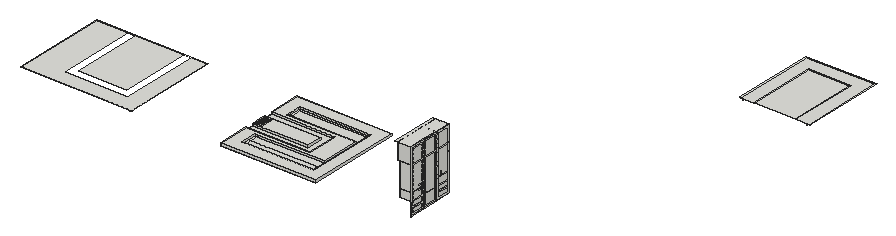
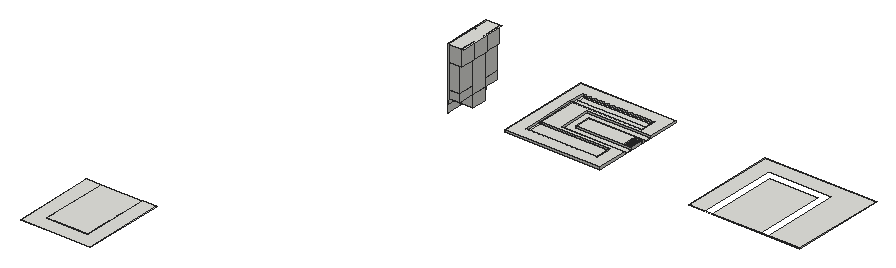
# SketchUp Ruby script. Lengths in inches.
U = 1.inch
M = Sketchup.active_model
def pt(a) = Geom::Point3d.new(a.map { |v| v * U })
def face(e, loops, mat)
  f = e.add_face(loops[0].map { |a| pt(a) })
  loops[1..].each { |l| e.add_face(l.map { |a| pt(a) }).erase! }
  f.material = f.back_material = mat if mat
  f
end
# faces: each face lists its corners as indices into pts; further lists are holes
def faces(e, pts, list, mat = nil) = list.each { |f| face(e, (f[0].is_a?(Array) ? f : [f]).map { |l| l.map { |i| pts[i] } }, mat) }
# xy, xz, yz: faces in a plane at the given z, y or x. An outline is a flat list of corners, or four numbers for a rectangle; further outlines are holes
def ring(l) = l.size == 4 ? [[l[0], l[1]], [l[2], l[1]], [l[2], l[3]], [l[0], l[3]]] : l.each_slice(2).to_a
def flat(e, list, mat, &to3) = list.each { |f| face(e, (f[0].is_a?(Array) ? f : [f]).map { |l| ring(l).map { |u, v| to3.(u, v) } }, mat) }
def xy(e, z, list, mat = nil) = flat(e, list, mat) { |x, y| [x, y, z] }
def xz(e, y, list, mat = nil) = flat(e, list, mat) { |x, z| [x, y, z] }
def yz(e, x, list, mat = nil) = flat(e, list, mat) { |y, z| [x, y, z] }
def lines(e, pts, list) = list.each { |a, b| e.add_line(pt(pts[a]), pt(pts[b])) }
# prism: a flat outline (further loops are holes) pulled along v
def prism(e, loops, v, mat = nil)
  f = face(e, loops, mat); d = Geom::Vector3d.new(v.map { |x| x * U })
  f.pushpull(f.normal.samedirection?(d) ? d.length : -d.length)
end
def box(e, o, s, mat = nil) = prism(e, [[o, [o[0] + s[0], o[1], o[2]], [o[0] + s[0], o[1] + s[1], o[2]], [o[0], o[1] + s[1], o[2]]]], [0, 0, s[2]], mat)
def at(x, y, z, deg = 0) = Geom::Transformation.translation(pt([x, y, z])) * Geom::Transformation.rotation(ORIGIN, Z_AXIS, deg.degrees)
def axes(o, x, y, z) = Geom::Transformation.new([*x, 0, *y, 0, *z, 0, *pt(o).to_a, 1])
def part(name) = M.definitions.add(name)
# library, detail: a bought-in or finely detailed component or shape, given as its bounding box
def library(name, o, s) = part(name).tap { |d| box(d.entities, o, s) }
def detail(e, o, s) = box(e.add_group.entities, o, s)
def put(e, d, t, mat = nil) = e.add_instance(d, t).tap { |i| i.material = mat if mat }
def group(e, t, mat = nil) = e.add_group.tap { |g| g.transformation = t; g.material = mat if mat }.entities
root = M.entities
xy(root,1.99,[[686.7,506.84,687.7,506.84,687.7,626.84,783.7,626.84,783.7,506.84,784.7,506.84,784.7,627.84,686.7,627.84]])
xy(root,3.49,[[682.7,506.84,683.7,506.84,683.7,630.84,787.7,630.84,787.7,506.84,788.7,506.84,788.7,631.84,682.7,631.84],[683.7,506.84,703.7,506.84,703.7,610.84,767.7,610.84,767.7,506.84,787.7,506.84,787.7,630.84,683.7,630.84],[703.7,506.84,704.7,506.84,704.7,609.84,766.7,609.84,766.7,506.84,767.7,506.84,767.7,610.84,703.7,610.84],[704.7,506.84,766.7,609.84]])
xy(root,4,[[539.16,65.91,557.16,89.16]])
xy(root,5,[[556.66,43.66,557.16,64.16],[556.66,90.91,557.16,112.16]])
xy(root,12,[[556.66,43.66,557.16,64.16],[556.66,90.91,557.16,112.16]])
xy(root,14,[[556.66,43.66,557.16,64.16],[556.28,90.91,557.16,112.16]])
xy(root,21,[[556.66,43.66,557.16,64.16],[556.28,90.91,557.16,112.16]])
xy(root,21.25,[[539.16,65.91,557.16,89.16]])
xy(root,22,[[539.16,42.66,557.16,65.16],[539.16,65.91,557.16,89.16],[539.16,89.91,557.16,113.16]])
xy(root,27.49,[[0,0,168,0,168,144,144,144,144,24,48,24,48,144,0,144],[303.04,0,447.04,144],[60,36,132,144]])
xy(root,27.98,[[321.04,18,429.04,18,429.04,30,426.04,30,426.04,21,324.04,21,324.04,30,321.04,30],[324.04,21,426.04,30],[321.04,30,324.04,42],[324.04,30,426.04,42],[426.04,30,429.04,42],
  [426.04,42,429.04,102],[303.04,48,399.04,48,399.04,96,303.04,96,303.04,84,387.04,84,387.04,60,303.04,60],[303.04,62.67,315.04,65.33],[303.04,68,315.04,70.67],[303.04,73.33,315.04,76],
  [303.04,78.67,315.04,81.33],[321.04,102,324.04,102,324.04,123,426.04,123,426.04,102,429.04,102,429.04,126,321.04,126],[324.04,102,426.04,123]])
xy(root,30.98,[[[303.04,0,447.04,0,447.04,144,303.04,144,303.04,96,399.04,96,399.04,48,303.04,48],[321.04,18,321.04,42,426.04,42,426.04,102,321.04,102,321.04,126,429.04,126,429.04,18]],[303.04,60,387.04,60,387.04,84,303.04,84,303.04,81.33,315.04,81.33,315.04,78.67,303.04,78.67,303.04,76,315.04,76,315.04,73.33,303.04,73.33,303.04,70.67,315.04,70.67,315.04,68,303.04,68,303.04,65.33,315.04,65.33,315.04,62.67,303.04,62.67]])
xy(root,33.25,[[539.16,42.66,557.16,65.16],[539.16,89.91,557.16,113.16]])
xy(root,34,[[539.16,42.66,557.16,65.16],[539.16,89.91,557.16,113.16]])
xy(root,70.5,[[539.16,42.66,557.16,65.16],[539.16,65.91,557.16,89.16],[539.16,89.91,557.16,113.16]])
xy(root,71.25,[[536.16,42.66,557.16,65.16],[536.16,65.91,557.16,89.16],[536.16,89.91,557.16,113.16]])
xy(root,95.25,[[536.16,42.66,557.16,65.16],[536.16,65.91,557.16,89.16],[536.16,89.91,557.16,113.16]])
xy(root,96,[[533.16,41.91,557.16,113.91]])
xz(root,0,[[0,27,168,27.49],[303.04,27.49,447.04,30.98]])
xz(root,18,[[321.04,27.98,429.04,30.98]])
xz(root,42,[[321.04,27.98,324.04,30.98],[324.04,27.98,426.04,30.98]])
xz(root,42.66,[[539.16,22,557.16,33.25],[539.16,34,557.16,70.5],[536.16,71.25,557.16,95.25]])
xz(root,43.66,[[556.66,5,557.16,12],[556.66,14,557.16,21]])
xz(root,48,[[303.04,27.98,399.04,30.98]])
xz(root,60,[[303.04,27.98,387.04,30.98]])
xz(root,62.67,[[303.04,27.98,315.04,30.98]])
xz(root,64.16,[[556.66,5,557.16,12],[556.66,14,557.16,21]])
xz(root,65.16,[[539.16,22,557.16,33.25],[539.16,34,557.16,70.5],[536.16,71.25,557.16,95.25]])
xz(root,65.33,[[303.04,27.98,315.04,30.98]])
xz(root,65.91,[[539.16,4,557.16,21.25],[539.16,22,557.16,70.5],[536.16,71.25,557.16,95.25]])
xz(root,68,[[303.04,27.98,315.04,30.98]])
xz(root,70.67,[[303.04,27.98,315.04,30.98]])
xz(root,73.33,[[303.04,27.98,315.04,30.98]])
xz(root,76,[[303.04,27.98,315.04,30.98]])
xz(root,78.67,[[303.04,27.98,315.04,30.98]])
xz(root,81.33,[[303.04,27.98,315.04,30.98]])
xz(root,84,[[303.04,27.98,387.04,30.98]])
xz(root,89.16,[[539.16,4,557.16,21.25],[539.16,22,557.16,70.5],[536.16,71.25,557.16,95.25]])
xz(root,89.91,[[539.16,22,557.16,33.25],[539.16,34,557.16,70.5],[536.16,71.25,557.16,95.25]])
xz(root,90.91,[[556.66,5,557.16,12],[556.28,14,557.16,21]])
xz(root,96,[[303.04,27.98,399.04,30.98]])
xz(root,102,[[321.04,27.98,324.04,30.98],[324.04,27.98,426.04,30.98]])
xz(root,112.16,[[556.66,5,557.16,12],[556.28,14,557.16,21]])
xz(root,113.16,[[539.16,22,557.16,33.25],[539.16,34,557.16,70.5],[536.16,71.25,557.16,95.25]])
xz(root,126,[[321.04,27.98,429.04,30.98]])
xz(root,144,[[0,27,168,27.49],[303.04,27.49,447.04,30.98]])
yz(root,0,[[0,27,144,27.49]])
yz(root,168,[[0,27,144,27.49]])
yz(root,303.04,[[0,27.49,0,30.98,48,30.98,48,27.98,60,27.98,60,30.98,62.67,30.98,62.67,27.98,65.33,27.98,65.33,30.98,68,30.98,68,27.98,70.67,27.98,70.67,30.98,73.33,30.98,73.33,27.98,76,27.98,76,30.98,78.67,30.98,78.67,27.98,81.33,27.98,81.33,30.98,84,30.98,84,27.98,96,27.98,96,30.98,144,30.98,144,27.49]])
yz(root,315.04,[[62.67,27.98,65.33,30.98],[68,27.98,70.67,30.98],[73.33,27.98,76,30.98],[78.67,27.98,81.33,30.98]])
yz(root,321.04,[[18,27.98,42,30.98],[102,27.98,126,30.98]])
yz(root,387.04,[[60,27.98,84,30.98]])
yz(root,399.04,[[48,27.98,96,30.98]])
yz(root,426.04,[[42,27.98,102,30.98]])
yz(root,429.04,[[18,27.98,42,30.98],[42,27.98,102,30.98],[102,27.98,126,30.98]])
yz(root,447.04,[[0,27.49,144,30.98]])
yz(root,536.16,[[42.66,71.25,65.16,95.25],[65.91,71.25,89.16,95.25],[89.91,71.25,113.16,95.25]])
yz(root,539.16,[[65.91,4,89.16,21.25],[42.66,22,65.16,33.25],[65.91,22,89.16,70.5],[89.91,22,113.16,33.25],[42.66,34,65.16,70.5],
  [89.91,34,113.16,70.5]])
yz(root,556.28,[[[90.91,14,112.16,21],[101.91,17,101.78,17.02,101.66,17.07,101.55,17.15,101.47,17.25,101.42,17.37,101.41,17.5,101.42,17.63,101.47,17.75,101.55,17.85,101.66,17.93,101.78,17.98,101.91,18,102.03,17.98,102.16,17.93,102.26,17.85,102.34,17.75,102.39,17.63,102.41,17.5,102.39,17.37,102.34,17.25,102.26,17.15,102.16,17.07,102.03,17.02]]])
yz(root,556.66,[[[43.66,5,64.16,12],[53.91,8,53.78,8.02,53.66,8.07,53.55,8.15,53.47,8.25,53.42,8.37,53.41,8.5,53.42,8.63,53.47,8.75,53.55,8.85,53.66,8.93,53.78,8.98,53.91,9,54.03,8.98,54.16,8.93,54.26,8.85,54.34,8.75,54.39,8.63,54.41,8.5,54.39,8.37,54.34,8.25,54.26,8.15,54.16,8.07,54.03,8.02]],[[90.91,5,112.16,12],[101.91,8,101.78,8.02,101.66,8.07,101.55,8.15,101.47,8.25,101.42,8.37,101.41,8.5,101.42,8.63,101.47,8.75,101.55,8.85,101.66,8.93,101.78,8.98,101.91,9,102.03,8.98,102.16,8.93,102.26,8.85,102.34,8.75,102.39,8.63,102.41,8.5,102.39,8.37,102.34,8.25,102.26,8.15,102.16,8.07,102.03,8.02]],[[43.66,14,64.16,21],[53.91,17,53.78,17.02,53.66,17.07,53.55,17.15,53.47,17.25,53.42,17.37,53.41,17.5,53.42,17.63,53.47,17.75,53.55,17.85,53.66,17.93,53.78,17.98,53.91,18,54.03,17.98,54.16,17.93,54.26,17.85,54.34,17.75,54.39,17.63,54.41,17.5,54.39,17.37,54.34,17.25,54.26,17.15,54.16,17.07,54.03,17.02]]])
yz(root,557.16,[[[42.66,4,65.16,13],[43.66,5,64.16,12]],[65.16,4,65.91,70.5],[89.16,4,89.91,70.5],[[89.91,4,113.16,13],[90.91,5,112.16,12]],[53.91,8,54.03,8.02,54.16,8.07,54.26,8.15,54.34,8.25,54.39,8.37,54.41,8.5,54.39,8.63,54.34,8.75,54.26,8.85,54.16,8.93,54.03,8.98,53.91,9,53.78,8.98,53.66,8.93,53.55,8.85,53.47,8.75,53.42,8.63,53.41,8.5,53.42,8.37,53.47,8.25,53.55,8.15,53.66,8.07,53.78,8.02],
  [101.91,8,102.03,8.02,102.16,8.07,102.26,8.15,102.34,8.25,102.39,8.37,102.41,8.5,102.39,8.63,102.34,8.75,102.26,8.85,102.16,8.93,102.03,8.98,101.91,9,101.78,8.98,101.66,8.93,101.55,8.85,101.47,8.75,101.42,8.63,101.41,8.5,101.42,8.37,101.47,8.25,101.55,8.15,101.66,8.07,101.78,8.02],[[42.66,13,65.16,22],[43.66,14,64.16,21]],[[89.91,13,113.16,22],[90.91,14,112.16,21]],[53.91,17,54.03,17.02,54.16,17.07,54.26,17.15,54.34,17.25,54.39,17.37,54.41,17.5,54.39,17.63,54.34,17.75,54.26,17.85,54.16,17.93,54.03,17.98,53.91,18,53.78,17.98,53.66,17.93,53.55,17.85,53.47,17.75,53.42,17.63,53.41,17.5,53.42,17.37,53.47,17.25,53.55,17.15,53.66,17.07,53.78,17.02],[101.91,17,102.03,17.02,102.16,17.07,102.26,17.15,102.34,17.25,102.39,17.37,102.41,17.5,102.39,17.63,102.34,17.75,102.26,17.85,102.16,17.93,102.03,17.98,101.91,18,101.78,17.98,101.66,17.93,101.55,17.85,101.47,17.75,101.42,17.63,101.41,17.5,101.42,17.37,101.47,17.25,101.55,17.15,101.66,17.07,101.78,17.02],
  [65.91,21.25,89.16,22],[42.66,33.25,65.16,34],[89.91,33.25,113.16,34],[42.66,70.5,113.16,71.25],[65.16,71.25,65.91,95.25],
  [89.16,71.25,89.91,95.25]])
p = [[557.16,53.78,8.02],[557.16,53.66,8.07],[556.66,53.66,8.07],[556.66,53.78,8.02],[557.16,53.91,8],[556.66,53.91,8],
  [557.16,54.03,8.02],[556.66,54.03,8.02],[557.16,54.16,8.07],[556.66,54.16,8.07],[557.16,101.78,8.02],[557.16,101.66,8.07],
  [556.66,101.66,8.07],[556.66,101.78,8.02],[557.16,101.91,8],[556.66,101.91,8],[557.16,102.03,8.02],[556.66,102.03,8.02],
  [557.16,102.16,8.07],[556.66,102.16,8.07],[557.16,53.55,8.15],[557.16,53.47,8.25],[556.66,53.47,8.25],[556.66,53.55,8.15],
  [557.16,54.26,8.15],[556.66,54.26,8.15],[557.16,54.34,8.25],[556.66,54.34,8.25],[557.16,101.55,8.15],[557.16,101.47,8.25],
  [556.66,101.47,8.25],[556.66,101.55,8.15],[557.16,102.26,8.15],[556.66,102.26,8.15],[557.16,102.34,8.25],[556.66,102.34,8.25],
  [557.16,53.42,8.37],[556.66,53.42,8.37],[557.16,54.39,8.37],[556.66,54.39,8.37],[557.16,101.42,8.37],[556.66,101.42,8.37],
  [557.16,102.39,8.37],[556.66,102.39,8.37],[557.16,53.41,8.5],[556.66,53.41,8.5],[557.16,54.41,8.5],[556.66,54.41,8.5],
  [557.16,101.41,8.5],[556.66,101.41,8.5],[557.16,102.41,8.5],[556.66,102.41,8.5],[557.16,53.42,8.63],[556.66,53.42,8.63],
  [557.16,54.39,8.63],[556.66,54.39,8.63],[557.16,101.42,8.63],[556.66,101.42,8.63],[557.16,102.39,8.63],[556.66,102.39,8.63],
  [557.16,53.47,8.75],[556.66,53.47,8.75],[557.16,54.34,8.75],[556.66,54.34,8.75],[557.16,101.47,8.75],[556.66,101.47,8.75],
  [557.16,102.34,8.75],[556.66,102.34,8.75],[557.16,53.55,8.85],[556.66,53.55,8.85],[557.16,54.26,8.85],[556.66,54.26,8.85],
  [557.16,101.55,8.85],[556.66,101.55,8.85],[557.16,102.26,8.85],[556.66,102.26,8.85],[557.16,53.66,8.93],[556.66,53.66,8.93],
  [557.16,53.78,8.98],[556.66,53.78,8.98],[557.16,54.03,8.98],[557.16,54.16,8.93],[556.66,54.16,8.93],[556.66,54.03,8.98],
  [557.16,101.66,8.93],[556.66,101.66,8.93],[557.16,101.78,8.98],[556.66,101.78,8.98],[557.16,102.03,8.98],[557.16,102.16,8.93],
  [556.66,102.16,8.93],[556.66,102.03,8.98],[557.16,53.91,9],[556.66,53.91,9],[557.16,101.91,9],[556.66,101.91,9],
  [557.16,53.78,17.02],[557.16,53.66,17.07],[556.66,53.66,17.07],[556.66,53.78,17.02],[557.16,53.91,17],[556.66,53.91,17],
  [557.16,54.03,17.02],[556.66,54.03,17.02],[557.16,54.16,17.07],[556.66,54.16,17.07],[557.16,101.78,17.02],[557.16,101.66,17.07],
  [556.28,101.66,17.07],[556.28,101.78,17.02],[557.16,101.91,17],[556.28,101.91,17],[557.16,102.03,17.02],[556.28,102.03,17.02],
  [557.16,102.16,17.07],[556.28,102.16,17.07],[557.16,53.55,17.15],[557.16,53.47,17.25],[556.66,53.47,17.25],[556.66,53.55,17.15],
  [557.16,54.26,17.15],[556.66,54.26,17.15],[557.16,54.34,17.25],[556.66,54.34,17.25],[557.16,101.55,17.15],[557.16,101.47,17.25],
  [556.28,101.47,17.25],[556.28,101.55,17.15],[557.16,102.26,17.15],[556.28,102.26,17.15],[557.16,102.34,17.25],[556.28,102.34,17.25],
  [557.16,53.42,17.37],[556.66,53.42,17.37],[557.16,54.39,17.37],[556.66,54.39,17.37],[557.16,101.42,17.37],[556.28,101.42,17.37],
  [557.16,102.39,17.37],[556.28,102.39,17.37],[557.16,53.41,17.5],[556.66,53.41,17.5],[557.16,54.41,17.5],[556.66,54.41,17.5],
  [557.16,101.41,17.5],[556.28,101.41,17.5],[557.16,102.41,17.5],[556.28,102.41,17.5],[557.16,53.42,17.63],[556.66,53.42,17.63],
  [557.16,54.39,17.63],[556.66,54.39,17.63],[557.16,101.42,17.63],[556.28,101.42,17.63],[557.16,102.39,17.63],[556.28,102.39,17.63],
  [557.16,53.47,17.75],[556.66,53.47,17.75],[557.16,54.34,17.75],[556.66,54.34,17.75],[557.16,101.47,17.75],[556.28,101.47,17.75],
  [557.16,102.34,17.75],[556.28,102.34,17.75],[557.16,53.55,17.85],[556.66,53.55,17.85],[557.16,54.26,17.85],[556.66,54.26,17.85],
  [557.16,101.55,17.85],[556.28,101.55,17.85],[557.16,102.26,17.85],[556.28,102.26,17.85],[557.16,53.66,17.93],[556.66,53.66,17.93],
  [557.16,53.78,17.98],[556.66,53.78,17.98],[557.16,54.03,17.98],[557.16,54.16,17.93],[556.66,54.16,17.93],[556.66,54.03,17.98],
  [557.16,101.66,17.93],[556.28,101.66,17.93],[557.16,101.78,17.98],[556.28,101.78,17.98],[557.16,102.03,17.98],[557.16,102.16,17.93],
  [556.28,102.16,17.93],[556.28,102.03,17.98],[557.16,53.91,18],[556.66,53.91,18],[557.16,101.91,18],[556.28,101.91,18]]
faces(root,p,[[0,1,2,3],[4,0,3,5],[6,4,5,7],[8,6,7,9],[10,11,12,13],[14,10,13,15],[16,14,15,17],[18,16,17,19],
  [20,21,22,23],[1,20,23,2],[24,8,9,25],[26,24,25,27],[28,29,30,31],[11,28,31,12],[32,18,19,33],[34,32,33,35],
  [21,36,37,22],[38,26,27,39],[29,40,41,30],[42,34,35,43],[36,44,45,37],[46,38,39,47],[40,48,49,41],[50,42,43,51],
  [44,52,53,45],[54,46,47,55],[48,56,57,49],[58,50,51,59],[52,60,61,53],[62,54,55,63],[56,64,65,57],[66,58,59,67],
  [60,68,69,61],[70,62,63,71],[64,72,73,65],[74,66,67,75],[68,76,77,69],[76,78,79,77],[80,81,82,83],[81,70,71,82],
  [72,84,85,73],[84,86,87,85],[88,89,90,91],[89,74,75,90],[78,92,93,79],[92,80,83,93],[86,94,95,87],[94,88,91,95],
  [96,97,98,99],[100,96,99,101],[102,100,101,103],[104,102,103,105],[106,107,108,109],[110,106,109,111],[112,110,111,113],[114,112,113,115],
  [116,117,118,119],[97,116,119,98],[120,104,105,121],[122,120,121,123],[124,125,126,127],[107,124,127,108],[128,114,115,129],[130,128,129,131],
  [117,132,133,118],[134,122,123,135],[125,136,137,126],[138,130,131,139],[132,140,141,133],[142,134,135,143],[136,144,145,137],[146,138,139,147],
  [140,148,149,141],[150,142,143,151],[144,152,153,145],[154,146,147,155],[148,156,157,149],[158,150,151,159],[152,160,161,153],[162,154,155,163],
  [156,164,165,157],[166,158,159,167],[160,168,169,161],[170,162,163,171],[164,172,173,165],[172,174,175,173],[176,177,178,179],[177,166,167,178],
  [168,180,181,169],[180,182,183,181],[184,185,186,187],[185,170,171,186],[174,188,189,175],[188,176,179,189],[182,190,191,183],[190,184,187,191]])
g1 = group(root,at(556.41,89.91,2))
xy(g1,0,[[0,0,0.75,24]])
xy(g1,94,[[0,0,0.75,24]])
xz(g1,0,[[0,0,0.75,94]])
xz(g1,24,[[0,0,0.75,94]])
yz(g1,0,[[0,0,24,94]])
yz(g1,0.75,[[[0,0,24,94],[1,1,23,93]],[[1,1,23,93],[3,3,21,91]],[[3,3,21,91],[7.0625,28.5625,9.3125,39]],[7.0625,28.5625,9.3125,39]])
g2 = group(root,at(556.41,65.91,2))
xy(g2,0,[[0,0,0.75,24]])
xy(g2,94,[[0,0,0.75,24]])
xz(g2,0,[[0,0,0.75,94]])
xz(g2,24,[[0,0,0.75,94]])
yz(g2,0,[[0,0,24,94]])
yz(g2,0.75,[[[0,0,24,94],[1,1,23,93]],[[1,1,23,93],[3,3,21,91]],[[3,3,21,91],[7,28.5625,9.25,39]],[7,28.5625,9.25,39]])
g3 = group(root,at(556.41,41.91,2))
xy(g3,0,[[0,0,0.75,24]])
xy(g3,94,[[0,0,0.75,24]])
xz(g3,0,[[0,0,0.75,94]])
xz(g3,24,[[0,0,0.75,94]])
yz(g3,0,[[0,0,24,94]])
yz(g3,0.75,[[[0,0,24,94],[1,1,23,93]],[[1,1,23,93],[3,3,21,91]],[[3,3,21,91],[14.75,28.5625,17,39]],[14.75,28.5625,17,39]])
